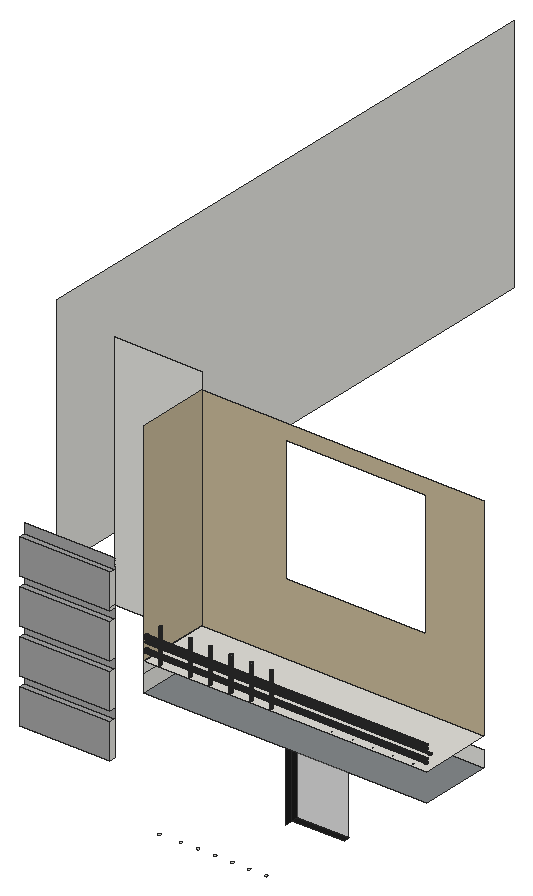
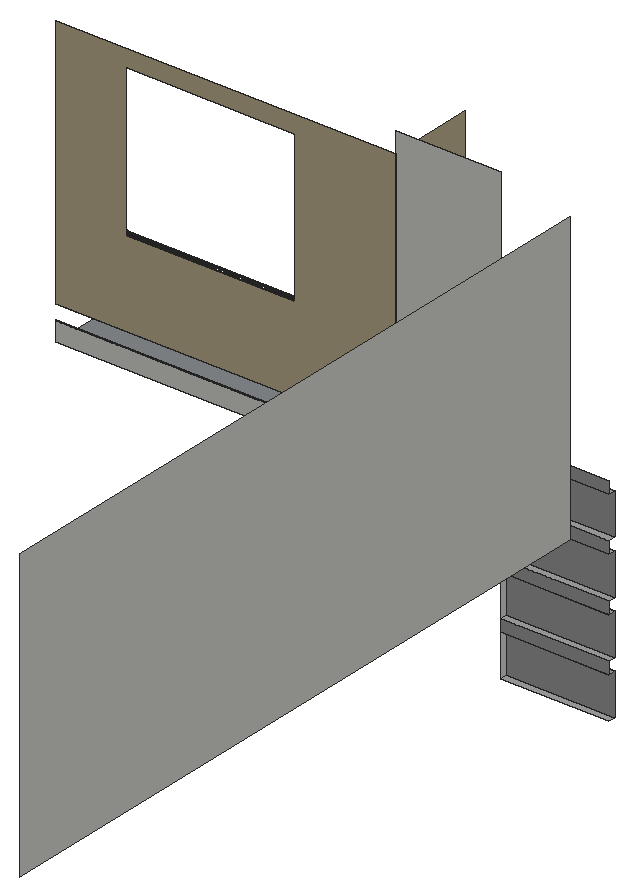
# SketchUp Ruby script. Lengths in inches.
U = 1.inch
M = Sketchup.active_model
def pt(a) = Geom::Point3d.new(a.map { |v| v * U })
def face(e, loops, mat)
  f = e.add_face(loops[0].map { |a| pt(a) })
  loops[1..].each { |l| e.add_face(l.map { |a| pt(a) }).erase! }
  f.material = f.back_material = mat if mat
  f
end
# faces: each face lists its corners as indices into pts; further lists are holes
def faces(e, pts, list, mat = nil) = list.each { |f| face(e, (f[0].is_a?(Array) ? f : [f]).map { |l| l.map { |i| pts[i] } }, mat) }
# xy, xz, yz: faces in a plane at the given z, y or x. An outline is a flat list of corners, or four numbers for a rectangle; further outlines are holes
def ring(l) = l.size == 4 ? [[l[0], l[1]], [l[2], l[1]], [l[2], l[3]], [l[0], l[3]]] : l.each_slice(2).to_a
def flat(e, list, mat, &to3) = list.each { |f| face(e, (f[0].is_a?(Array) ? f : [f]).map { |l| ring(l).map { |u, v| to3.(u, v) } }, mat) }
def xy(e, z, list, mat = nil) = flat(e, list, mat) { |x, y| [x, y, z] }
def xz(e, y, list, mat = nil) = flat(e, list, mat) { |x, z| [x, y, z] }
def yz(e, x, list, mat = nil) = flat(e, list, mat) { |y, z| [x, y, z] }
def lines(e, pts, list) = list.each { |a, b| e.add_line(pt(pts[a]), pt(pts[b])) }
# prism: a flat outline (further loops are holes) pulled along v
def prism(e, loops, v, mat = nil)
  f = face(e, loops, mat); d = Geom::Vector3d.new(v.map { |x| x * U })
  f.pushpull(f.normal.samedirection?(d) ? d.length : -d.length)
end
def box(e, o, s, mat = nil) = prism(e, [[o, [o[0] + s[0], o[1], o[2]], [o[0] + s[0], o[1] + s[1], o[2]], [o[0], o[1] + s[1], o[2]]]], [0, 0, s[2]], mat)
def at(x, y, z, deg = 0) = Geom::Transformation.translation(pt([x, y, z])) * Geom::Transformation.rotation(ORIGIN, Z_AXIS, deg.degrees)
def axes(o, x, y, z) = Geom::Transformation.new([*x, 0, *y, 0, *z, 0, *pt(o).to_a, 1])
def part(name) = M.definitions.add(name)
# library, detail: a bought-in or finely detailed component or shape, given as its bounding box
def library(name, o, s) = part(name).tap { |d| box(d.entities, o, s) }
def detail(e, o, s) = box(e.add_group.entities, o, s)
def put(e, d, t, mat = nil) = e.add_instance(d, t).tap { |i| i.material = mat if mat }
def group(e, t, mat = nil) = e.add_group.tap { |g| g.transformation = t; g.material = mat if mat }.entities
root = M.entities
M.materials.add("[0133_Gray]").color = [128, 128, 128]
M.materials.add("[Blacktop New]").color = [30, 30, 30]
M.materials.add("[Blacktop Old 01]").color = [132, 136, 139]
M.materials.add("[Marble Carrara Gold Floor Tile]").color = [225, 223, 217]
M.materials.add("[Pavers Flagstone Gray]").color = [162, 162, 162]
M.materials.add("[Quartz Light Brown]").color = [199, 184, 152]
M.materials.add("[Translucent Glass Gray]").color = [128, 128, 128]
M.materials["[Translucent Glass Gray]"].alpha = 0.5
xy(root,170.4,[[95.31,3.4,95.45,3.4,95.57,3.44,95.68,3.52,95.76,3.61,95.82,3.73,95.85,3.86,95.84,3.99,95.8,4.11,95.73,4.22,95.63,4.31,95.51,4.37,95.39,4.39,95.26,4.39,95.13,4.34,95.02,4.27,94.9375,4.18,94.88,4.06,94.85,3.93,94.86,3.8,94.9,3.68,94.97,3.57,95.07,3.48,95.1875,3.42]])
xy(root,170.77,[[106.13,3.4,106.26,3.4,106.38,3.44,106.49,3.52,106.58,3.61,106.64,3.73,106.66,3.86,106.65,3.99,106.61,4.11,106.54,4.22,106.44,4.31,106.33,4.37,106.2,4.39,106.07,4.39,105.94,4.34,105.84,4.27,105.75,4.18,105.69,4.06,105.66,3.93,105.67,3.8,105.71,3.68,105.79,3.57,105.88,3.48,106,3.42],[114.69,3.4,114.82,3.4,114.94,3.44,115.05,3.52,115.14,3.61,115.2,3.73,115.22,3.86,115.22,3.99,115.18,4.11,115.1,4.22,115.01,4.31,114.89,4.37,114.76,4.39,114.63,4.39,114.51,4.34,114.4,4.27,114.3125,4.18,114.25,4.06,114.23,3.93,114.23,3.8,114.28,3.68,114.35,3.57,114.45,3.48,114.5625,3.42],[123.25,3.4,123.38,3.4,123.51,3.44,123.62,3.52,123.7,3.61,123.76,3.73,123.79,3.86,123.78,3.99,123.74,4.11,123.67,4.22,123.57,4.31,123.45,4.37,123.32,4.39,123.19,4.39,123.07,4.34,122.96,4.27,122.875,4.18,122.82,4.06,122.79,3.93,122.8,3.8,122.84,3.68,122.91,3.57,123.01,3.48,123.125,3.42],[131.81,3.4,131.95,3.4,132.07,3.44,132.18,3.52,132.26,3.61,132.32,3.73,132.35,3.86,132.34,3.99,132.3,4.11,132.23,4.22,132.13,4.31,132.01,4.37,131.89,4.39,131.76,4.39,131.63,4.34,131.52,4.27,131.4375,4.18,131.38,4.06,131.35,3.93,131.36,3.8,131.4,3.68,131.47,3.57,131.57,3.48,131.6875,3.42],[140.38,3.4,140.51,3.4,140.63,3.44,140.74,3.52,140.83,3.61,140.89,3.73,140.91,3.86,140.9,3.99,140.86,4.11,140.79,4.22,140.69,4.31,140.58,4.37,140.45,4.39,140.32,4.39,140.19,4.34,140.09,4.27,140,4.18,139.94,4.06,139.91,3.93,139.92,3.8,139.96,3.68,140.04,3.57,140.13,3.48,140.25,3.42],
  [148.94,3.4,149.07,3.4,149.19,3.44,149.3,3.52,149.39,3.61,149.45,3.73,149.47,3.86,149.47,3.99,149.43,4.11,149.35,4.22,149.26,4.31,149.14,4.37,149.01,4.39,148.88,4.39,148.76,4.34,148.65,4.27,148.5625,4.18,148.5,4.06,148.48,3.93,148.48,3.8,148.53,3.68,148.6,3.57,148.7,3.48,148.8125,3.42]])
xy(root,171.57,[[0,36,45.0625,39]],"[Pavers Flagstone Gray]")
xy(root,176.78,[[136.06,36,162.28,39]],"[Blacktop New]")
xy(root,188.9375,[[0,36,45.0625,39]],"[Pavers Flagstone Gray]")
xy(root,193.95,[[0,36,45.0625,39]],"[Pavers Flagstone Gray]")
xy(root,211.3125,[[0,36,45.0625,39]],"[Pavers Flagstone Gray]")
xy(root,216.32,[[0,36,45.0625,39]],"[Pavers Flagstone Gray]")
xy(root,220.84,[[136.06,36,162.28,39]],"[Blacktop New]")
xy(root,232,[[88.53,3,229.62,39]],"[Blacktop Old 01]")
xy(root,233.6875,[[0,36,45.0625,39]],"[Pavers Flagstone Gray]")
xy(root,238.7,[[0,36,45.0625,39]],"[Pavers Flagstone Gray]")
xy(root,246.23,[[[88.53,3,229.62,39],[110.48,3.83,110.32,3.85,110.17,3.92,110.04,4.02,109.9375,4.15,109.875,4.3,109.85,4.46,109.875,4.62,109.9375,4.77,110.04,4.9,110.17,5,110.32,5.0625,110.48,5.08,110.64,5.0625,110.79,5,110.92,4.9,111.02,4.77,111.08,4.62,111.1,4.46,111.08,4.3,111.02,4.15,110.92,4.02,110.79,3.92,110.64,3.85],[120.6,3.83,120.44,3.85,120.29,3.92,120.16,4.02,120.0625,4.15,120,4.3,119.98,4.46,120,4.62,120.0625,4.77,120.16,4.9,120.29,5,120.44,5.0625,120.6,5.08,120.77,5.0625,120.92,5,121.05,4.9,121.15,4.77,121.21,4.62,121.23,4.46,121.21,4.3,121.15,4.15,121.05,4.02,120.92,3.92,120.77,3.85],[130.73,3.83,130.57,3.85,130.42,3.92,130.29,4.02,130.1875,4.15,130.125,4.3,130.1,4.46,130.125,4.62,130.1875,4.77,130.29,4.9,130.42,5,130.57,5.0625,130.73,5.08,130.89,5.0625,131.04,5,131.17,4.9,131.27,4.77,131.33,4.62,131.35,4.46,131.33,4.3,131.27,4.15,131.17,4.02,131.04,3.92,130.89,3.85],[140.85,3.83,140.69,3.85,140.54,3.92,140.41,4.02,140.3125,4.15,140.25,4.3,140.23,4.46,140.25,4.62,140.3125,4.77,140.41,4.9,140.54,5,140.69,5.0625,140.85,5.08,141.02,5.0625,141.17,5,141.3,4.9,141.4,4.77,141.46,4.62,141.48,4.46,141.46,4.3,141.4,4.15,141.3,4.02,141.17,3.92,141.02,3.85],[150.98,3.83,150.82,3.85,150.67,3.92,150.54,4.02,150.4375,4.15,150.375,4.3,150.35,4.46,150.375,4.62,150.4375,4.77,150.54,4.9,150.67,5,150.82,5.0625,150.98,5.08,151.14,5.0625,151.29,5,151.42,4.9,151.52,4.77,151.58,4.62,151.6,4.46,151.58,4.3,151.52,4.15,151.42,4.02,151.29,3.92,151.14,3.85],[161.1,3.83,160.94,3.85,160.79,3.92,160.66,4.02,160.5625,4.15,160.5,4.3,160.48,4.46,160.5,4.62,160.5625,4.77,160.66,4.9,160.79,5,160.94,5.0625,161.1,5.08,161.27,5.0625,161.42,5,161.55,4.9,161.65,4.77,161.71,4.62,161.73,4.46,161.71,4.3,161.65,4.15,161.55,4.02,161.42,3.92,161.27,3.85],[171.23,3.83,171.07,3.85,170.92,3.92,170.79,4.02,170.6875,4.15,170.625,4.3,170.6,4.46,170.625,4.62,170.6875,4.77,170.79,4.9,170.92,5,171.07,5.0625,171.23,5.08,171.39,5.0625,171.54,5,171.67,4.9,171.77,4.77,171.83,4.62,171.85,4.46,171.83,4.3,171.77,4.15,171.67,4.02,171.54,3.92,171.39,3.85],[181.35,3.83,181.19,3.85,181.04,3.92,180.91,4.02,180.8125,4.15,180.75,4.3,180.73,4.46,180.75,4.62,180.8125,4.77,180.91,4.9,181.04,5,181.19,5.0625,181.35,5.08,181.52,5.0625,181.67,5,181.8,4.9,181.9,4.77,181.96,4.62,181.98,4.46,181.96,4.3,181.9,4.15,181.8,4.02,181.67,3.92,181.52,3.85],[95.48,3.83,95.32,3.85,95.17,3.92,95.04,4.02,94.9375,4.15,94.875,4.3,94.85,4.46,94.875,4.62,94.9375,4.77,95.04,4.9,95.17,5,95.32,5.0625,95.48,5.08,95.64,5.0625,95.79,5,95.92,4.9,96.02,4.77,96.08,4.62,96.1,4.46,96.08,4.3,96.02,4.15,95.92,4.02,95.79,3.92,95.64,3.85],[191.48,3.83,191.32,3.85,191.17,3.92,191.04,4.02,190.9375,4.15,190.875,4.3,190.85,4.46,190.875,4.62,190.9375,4.77,191.04,4.9,191.17,5,191.32,5.0625,191.48,5.08,191.64,5.0625,191.79,5,191.92,4.9,192.02,4.77,192.08,4.62,192.1,4.46,192.08,4.3,192.02,4.15,191.92,4.02,191.79,3.92,191.64,3.85],[201.6,3.83,201.44,3.85,201.29,3.92,201.16,4.02,201.0625,4.15,201,4.3,200.98,4.46,201,4.62,201.0625,4.77,201.16,4.9,201.29,5,201.44,5.0625,201.6,5.08,201.77,5.0625,201.92,5,202.05,4.9,202.15,4.77,202.21,4.62,202.23,4.46,202.21,4.3,202.15,4.15,202.05,4.02,201.92,3.92,201.77,3.85],[211.73,3.83,211.57,3.85,211.42,3.92,211.29,4.02,211.1875,4.15,211.125,4.3,211.1,4.46,211.125,4.62,211.1875,4.77,211.29,4.9,211.42,5,211.57,5.0625,211.73,5.08,211.89,5.0625,212.04,5,212.17,4.9,212.27,4.77,212.33,4.62,212.35,4.46,212.33,4.3,212.27,4.15,212.17,4.02,212.04,3.92,211.89,3.85],[221.85,3.83,221.69,3.85,221.54,3.92,221.41,4.02,221.3125,4.15,221.25,4.3,221.23,4.46,221.25,4.62,221.3125,4.77,221.41,4.9,221.54,5,221.69,5.0625,221.85,5.08,222.02,5.0625,222.17,5,222.3,4.9,222.4,4.77,222.46,4.62,222.48,4.46,222.46,4.3,222.4,4.15,222.3,4.02,222.17,3.92,222.02,3.85]]],"[Marble Carrara Gold Floor Tile]")
xy(root,256.0625,[[0,36,45.0625,39]],"[Pavers Flagstone Gray]")
xz(root,36,[[0,171.57,45.0625,188.9375],[0,193.95,45.0625,211.3125],[0,216.32,45.0625,233.6875],[0,238.7,45.0625,256.0625]],"[Pavers Flagstone Gray]")
xz(root,39,[[88.53,232,229.62,240],[45.0625,240,88.53,360],[88.53,240,229.62,240.1875]])
xz(root,39,[[0,188.9375,45.0625,193.95],[0,211.3125,45.0625,216.32],[0,233.6875,45.0625,238.7],[0,256.0625,45.0625,261.07]],"[Pavers Flagstone Gray]")
xz(root,39,[[[88.53,246.23,229.62,351.5625],[130.59,281.71,200.77,344.28]]],"[Quartz Light Brown]")
xz(root,39,[[136.06,176.78,162.28,220.84]],"[Translucent Glass Gray]")
yz(root,9,[[48,240,333.4375,360]])
yz(root,45.0625,[[36,171.57,39,188.9375],[36,193.95,39,211.3125],[36,216.32,39,233.6875],[36,238.7,39,240],[36,240,39,256.0625]])
yz(root,88.53,[[3,232,39,240.1875],[3,240.1875,39,246.23]])
yz(root,88.53,[[[3,246.23,39,351.5625],[3.53,257.33,3.43,257.34,3.34,257.375,3.26,257.43,3.2,257.51,3.16,257.6,3.15,257.7,3.16,257.8,3.2,257.89,3.26,257.97,3.34,258.02,3.43,258.0625,3.53,258.08,3.625,258.0625,3.71,258.02,3.79,257.97,3.85,257.89,3.89,257.8,3.9,257.7,3.89,257.6,3.85,257.51,3.79,257.43,3.71,257.375,3.625,257.34],[3.53,258.89,3.43,258.9,3.34,258.9375,3.26,259,3.2,259.08,3.16,259.17,3.15,259.26,3.16,259.36,3.2,259.45,3.26,259.53,3.34,259.59,3.43,259.625,3.53,259.64,3.625,259.625,3.71,259.59,3.79,259.53,3.85,259.45,3.89,259.36,3.9,259.26,3.89,259.17,3.85,259.08,3.79,259,3.71,258.9375,3.625,258.9],[3.53,260.45,3.43,260.46,3.34,260.5,3.26,260.56,3.2,260.64,3.16,260.73,3.15,260.83,3.16,260.92,3.2,261.01,3.26,261.09,3.34,261.15,3.43,261.1875,3.53,261.2,3.625,261.1875,3.71,261.15,3.79,261.09,3.85,261.01,3.89,260.92,3.9,260.83,3.89,260.73,3.85,260.64,3.79,260.56,3.71,260.5,3.625,260.46],[3.53,262.01,3.43,262.03,3.34,262.0625,3.26,262.12,3.2,262.2,3.16,262.29,3.15,262.39,3.16,262.48,3.2,262.58,3.26,262.65,3.34,262.71,3.43,262.75,3.53,262.76,3.625,262.75,3.71,262.71,3.79,262.65,3.85,262.58,3.89,262.48,3.9,262.39,3.89,262.29,3.85,262.2,3.79,262.12,3.71,262.0625,3.625,262.03],[3.53,255.76,3.43,255.78,3.34,255.8125,3.26,255.87,3.2,255.95,3.16,256.04,3.15,256.14,3.16,256.23,3.2,256.33,3.26,256.4,3.34,256.46,3.43,256.5,3.53,256.51,3.625,256.5,3.71,256.46,3.79,256.4,3.85,256.33,3.89,256.23,3.9,256.14,3.89,256.04,3.85,255.95,3.79,255.87,3.71,255.8125,3.625,255.78],[3.53,247.95,3.43,247.96,3.34,248,3.26,248.06,3.2,248.14,3.16,248.23,3.15,248.33,3.16,248.42,3.2,248.51,3.26,248.59,3.34,248.65,3.43,248.6875,3.53,248.7,3.625,248.6875,3.71,248.65,3.79,248.59,3.85,248.51,3.89,248.42,3.9,248.33,3.89,248.23,3.85,248.14,3.79,248.06,3.71,248,3.625,247.96],[3.53,249.51,3.43,249.53,3.34,249.5625,3.26,249.62,3.2,249.7,3.16,249.79,3.15,249.89,3.16,249.98,3.2,250.08,3.26,250.15,3.34,250.21,3.43,250.25,3.53,250.26,3.625,250.25,3.71,250.21,3.79,250.15,3.85,250.08,3.89,249.98,3.9,249.89,3.89,249.79,3.85,249.7,3.79,249.62,3.71,249.5625,3.625,249.53],[3.53,251.08,3.43,251.09,3.34,251.125,3.26,251.18,3.2,251.26,3.16,251.35,3.15,251.45,3.16,251.55,3.2,251.64,3.26,251.72,3.34,251.77,3.43,251.8125,3.53,251.83,3.625,251.8125,3.71,251.77,3.79,251.72,3.85,251.64,3.89,251.55,3.9,251.45,3.89,251.35,3.85,251.26,3.79,251.18,3.71,251.125,3.625,251.09],[3.53,252.64,3.43,252.65,3.34,252.6875,3.26,252.75,3.2,252.83,3.16,252.92,3.15,253.01,3.16,253.11,3.2,253.2,3.26,253.28,3.34,253.34,3.43,253.375,3.53,253.39,3.625,253.375,3.71,253.34,3.79,253.28,3.85,253.2,3.89,253.11,3.9,253.01,3.89,252.92,3.85,252.83,3.79,252.75,3.71,252.6875,3.625,252.65],[3.53,254.2,3.43,254.21,3.34,254.25,3.26,254.31,3.2,254.39,3.16,254.48,3.15,254.58,3.16,254.67,3.2,254.76,3.26,254.84,3.34,254.9,3.43,254.9375,3.53,254.95,3.625,254.9375,3.71,254.9,3.79,254.84,3.85,254.76,3.89,254.67,3.9,254.58,3.89,254.48,3.85,254.39,3.79,254.31,3.71,254.25,3.625,254.21]]],"[Quartz Light Brown]")
yz(root,133.06,[[36,173.78,39,223.84]],"[Blacktop New]")
yz(root,136.06,[[36,176.78,39,220.84]],"[Blacktop New]")
p = [[95.32,3.85,246.23],[95.48,3.83,246.23],[95.48,3.83,263.16],[95.32,3.85,263.16],[95.64,3.85,246.23],[95.64,3.85,263.16],
  [110.32,3.85,246.23],[110.48,3.83,246.23],[110.48,3.83,263.16],[110.32,3.85,263.16],[110.64,3.85,246.23],[110.64,3.85,263.16],
  [120.44,3.85,246.23],[120.6,3.83,246.23],[120.6,3.83,263.16],[120.44,3.85,263.16],[120.77,3.85,246.23],[120.77,3.85,263.16],
  [130.57,3.85,246.23],[130.73,3.83,246.23],[130.73,3.83,263.16],[130.57,3.85,263.16],[130.89,3.85,246.23],[130.89,3.85,263.16],
  [140.69,3.85,246.23],[140.85,3.83,246.23],[140.85,3.83,263.16],[140.69,3.85,263.16],[141.02,3.85,246.23],[141.02,3.85,263.16],
  [150.82,3.85,246.23],[150.98,3.83,246.23],[150.98,3.83,263.16],[150.82,3.85,263.16],[151.14,3.85,246.23],[151.14,3.85,263.16],
  [95.04,4.02,246.23],[95.17,3.92,246.23],[95.17,3.92,263.16],[95.04,4.02,263.16],[95.79,3.92,246.23],[95.79,3.92,263.16],
  [95.92,4.02,246.23],[95.92,4.02,263.16],[110.04,4.02,246.23],[110.17,3.92,246.23],[110.17,3.92,263.16],[110.04,4.02,263.16],
  [110.79,3.92,246.23],[110.79,3.92,263.16],[110.92,4.02,246.23],[110.92,4.02,263.16],[120.16,4.02,246.23],[120.29,3.92,246.23],
  [120.29,3.92,263.16],[120.16,4.02,263.16],[120.92,3.92,246.23],[120.92,3.92,263.16],[121.05,4.02,246.23],[121.05,4.02,263.16],
  [130.29,4.02,246.23],[130.42,3.92,246.23],[130.42,3.92,263.16],[130.29,4.02,263.16],[131.04,3.92,246.23],[131.04,3.92,263.16],
  [131.17,4.02,246.23],[131.17,4.02,263.16],[140.41,4.02,246.23],[140.54,3.92,246.23],[140.54,3.92,263.16],[140.41,4.02,263.16],
  [141.17,3.92,246.23],[141.17,3.92,263.16],[141.3,4.02,246.23],[141.3,4.02,263.16],[150.54,4.02,246.23],[150.67,3.92,246.23],
  [150.67,3.92,263.16],[150.54,4.02,263.16],[151.29,3.92,246.23],[151.29,3.92,263.16],[151.42,4.02,246.23],[151.42,4.02,263.16],
  [94.9375,4.15,246.23],[94.9375,4.15,263.16],[96.02,4.15,246.23],[96.02,4.15,263.16],[109.9375,4.15,246.23],[109.9375,4.15,263.16],
  [111.02,4.15,246.23],[111.02,4.15,263.16],[120.0625,4.15,246.23],[120.0625,4.15,263.16],[121.15,4.15,246.23],[121.15,4.15,263.16],
  [130.1875,4.15,246.23],[130.1875,4.15,263.16],[131.27,4.15,246.23],[131.27,4.15,263.16],[140.3125,4.15,246.23],[140.3125,4.15,263.16],
  [141.4,4.15,246.23],[141.4,4.15,263.16],[150.4375,4.15,246.23],[150.4375,4.15,263.16],[151.52,4.15,246.23],[151.52,4.15,263.16],
  [94.875,4.3,246.23],[94.875,4.3,263.16],[96.08,4.3,246.23],[96.08,4.3,263.16],[109.875,4.3,246.23],[109.875,4.3,263.16],
  [111.08,4.3,246.23],[111.08,4.3,263.16],[120,4.3,246.23],[120,4.3,263.16],[121.21,4.3,246.23],[121.21,4.3,263.16],
  [130.125,4.3,246.23],[130.125,4.3,263.16],[131.33,4.3,246.23],[131.33,4.3,263.16],[140.25,4.3,246.23],[140.25,4.3,263.16],
  [141.46,4.3,246.23],[141.46,4.3,263.16],[150.375,4.3,246.23],[150.375,4.3,263.16],[151.58,4.3,246.23],[151.58,4.3,263.16],
  [94.85,4.46,246.23],[94.85,4.46,263.16],[96.1,4.46,246.23],[96.1,4.46,263.16],[109.85,4.46,246.23],[109.85,4.46,263.16],
  [111.1,4.46,246.23],[111.1,4.46,263.16],[119.98,4.46,246.23],[119.98,4.46,263.16],[121.23,4.46,246.23],[121.23,4.46,263.16],
  [130.1,4.46,246.23],[130.1,4.46,263.16],[131.35,4.46,246.23],[131.35,4.46,263.16],[140.23,4.46,246.23],[140.23,4.46,263.16],
  [141.48,4.46,246.23],[141.48,4.46,263.16],[150.35,4.46,246.23],[150.35,4.46,263.16],[151.6,4.46,246.23],[151.6,4.46,263.16],
  [94.875,4.62,246.23],[94.875,4.62,263.16],[96.08,4.62,246.23],[96.08,4.62,263.16],[109.875,4.62,246.23],[109.875,4.62,263.16],
  [111.08,4.62,246.23],[111.08,4.62,263.16],[120,4.62,246.23],[120,4.62,263.16],[121.21,4.62,246.23],[121.21,4.62,263.16],
  [130.125,4.62,246.23],[130.125,4.62,263.16],[131.33,4.62,246.23],[131.33,4.62,263.16],[140.25,4.62,246.23],[140.25,4.62,263.16],
  [141.46,4.62,246.23],[141.46,4.62,263.16],[150.375,4.62,246.23],[150.375,4.62,263.16],[151.58,4.62,246.23],[151.58,4.62,263.16],
  [94.9375,4.77,246.23],[94.9375,4.77,263.16],[96.02,4.77,246.23],[96.02,4.77,263.16],[109.9375,4.77,246.23],[109.9375,4.77,263.16],
  [111.02,4.77,246.23],[111.02,4.77,263.16],[120.0625,4.77,246.23],[120.0625,4.77,263.16],[121.15,4.77,246.23],[121.15,4.77,263.16],
  [130.1875,4.77,246.23],[130.1875,4.77,263.16],[131.27,4.77,246.23],[131.27,4.77,263.16],[140.3125,4.77,246.23],[140.3125,4.77,263.16],
  [141.4,4.77,246.23],[141.4,4.77,263.16],[150.4375,4.77,246.23],[150.4375,4.77,263.16],[151.52,4.77,246.23],[151.52,4.77,263.16],
  [95.04,4.9,246.23],[95.04,4.9,263.16],[95.92,4.9,246.23],[95.92,4.9,263.16],[110.04,4.9,246.23],[110.04,4.9,263.16],
  [110.92,4.9,246.23],[110.92,4.9,263.16],[120.16,4.9,246.23],[120.16,4.9,263.16],[121.05,4.9,246.23],[121.05,4.9,263.16],
  [130.29,4.9,246.23],[130.29,4.9,263.16],[131.17,4.9,246.23],[131.17,4.9,263.16],[140.41,4.9,246.23],[140.41,4.9,263.16],
  [141.3,4.9,246.23],[141.3,4.9,263.16],[150.54,4.9,246.23],[150.54,4.9,263.16],[151.42,4.9,246.23],[151.42,4.9,263.16],
  [95.17,5,246.23],[95.17,5,263.16],[95.79,5,246.23],[95.79,5,263.16],[110.17,5,246.23],[110.17,5,263.16],
  [110.79,5,246.23],[110.79,5,263.16],[120.29,5,246.23],[120.29,5,263.16],[120.92,5,246.23],[120.92,5,263.16],
  [130.42,5,246.23],[130.42,5,263.16],[131.04,5,246.23],[131.04,5,263.16],[140.54,5,246.23],[140.54,5,263.16],
  [141.17,5,246.23],[141.17,5,263.16],[150.67,5,246.23],[150.67,5,263.16],[151.29,5,246.23],[151.29,5,263.16],
  [95.32,5.0625,246.23],[95.32,5.0625,263.16],[95.64,5.0625,246.23],[95.64,5.0625,263.16],[110.32,5.0625,246.23],[110.32,5.0625,263.16],
  [110.64,5.0625,246.23],[110.64,5.0625,263.16],[120.44,5.0625,246.23],[120.44,5.0625,263.16],[120.77,5.0625,246.23],[120.77,5.0625,263.16],
  [130.57,5.0625,246.23],[130.57,5.0625,263.16],[130.89,5.0625,246.23],[130.89,5.0625,263.16],[140.69,5.0625,246.23],[140.69,5.0625,263.16],
  [141.02,5.0625,246.23],[141.02,5.0625,263.16],[150.82,5.0625,246.23],[150.82,5.0625,263.16],[151.14,5.0625,246.23],[151.14,5.0625,263.16],
  [95.48,5.08,246.23],[95.48,5.08,263.16],[110.48,5.08,246.23],[110.48,5.08,263.16],[120.6,5.08,246.23],[120.6,5.08,263.16],
  [130.73,5.08,246.23],[130.73,5.08,263.16],[140.85,5.08,246.23],[140.85,5.08,263.16],[150.98,5.08,246.23],[150.98,5.08,263.16],
  [88.53,3.34,249.5625],[88.53,3.43,249.53],[229.62,3.43,249.53],[229.62,3.34,249.5625],[88.53,3.53,249.51],[229.62,3.53,249.51],
  [88.53,3.625,249.53],[229.62,3.625,249.53],[88.53,3.71,249.5625],[229.62,3.71,249.5625],[88.53,3.2,249.7],[88.53,3.26,249.62],
  [229.62,3.26,249.62],[229.62,3.2,249.7],[88.53,3.79,249.62],[229.62,3.79,249.62],[88.53,3.85,249.7],[229.62,3.85,249.7],
  [88.53,3.16,249.79],[229.62,3.16,249.79],[88.53,3.89,249.79],[229.62,3.89,249.79],[88.53,3.15,249.89],[229.62,3.15,249.89],
  [88.53,3.9,249.89],[229.62,3.9,249.89],[88.53,3.16,249.98],[229.62,3.16,249.98],[88.53,3.89,249.98],[229.62,3.89,249.98],
  [88.53,3.2,250.08],[229.62,3.2,250.08],[88.53,3.85,250.08],[229.62,3.85,250.08],[88.53,3.26,250.15],[229.62,3.26,250.15],
  [88.53,3.79,250.15],[229.62,3.79,250.15],[88.53,3.34,250.21],[229.62,3.34,250.21],[88.53,3.43,250.25],[229.62,3.43,250.25],
  [88.53,3.53,250.26],[229.62,3.53,250.26],[88.53,3.625,250.25],[229.62,3.625,250.25],[88.53,3.71,250.21],[229.62,3.71,250.21],
  [88.53,3.34,251.125],[88.53,3.43,251.09],[229.62,3.43,251.09],[229.62,3.34,251.125],[88.53,3.26,251.18],[229.62,3.26,251.18],
  [88.53,3.53,251.08],[229.62,3.53,251.08],[88.53,3.625,251.09],[229.62,3.625,251.09],[88.53,3.71,251.125],[229.62,3.71,251.125],
  [88.53,3.79,251.18],[229.62,3.79,251.18],[88.53,3.2,251.26],[229.62,3.2,251.26],[88.53,3.85,251.26],[229.62,3.85,251.26],
  [88.53,3.16,251.35],[229.62,3.16,251.35],[88.53,3.89,251.35],[229.62,3.89,251.35],[88.53,3.15,251.45],[229.62,3.15,251.45],
  [88.53,3.9,251.45],[229.62,3.9,251.45],[88.53,3.16,251.55],[229.62,3.16,251.55],[88.53,3.2,251.64],[229.62,3.2,251.64],
  [88.53,3.89,251.55],[229.62,3.89,251.55],[88.53,3.85,251.64],[229.62,3.85,251.64],[88.53,3.26,251.72],[229.62,3.26,251.72],
  [88.53,3.79,251.72],[229.62,3.79,251.72],[88.53,3.34,251.77],[229.62,3.34,251.77],[88.53,3.71,251.77],[229.62,3.71,251.77],
  [88.53,3.43,251.8125],[229.62,3.43,251.8125],[88.53,3.53,251.83],[229.62,3.53,251.83],[88.53,3.625,251.8125],[229.62,3.625,251.8125],
  [88.53,3.34,254.25],[88.53,3.43,254.21],[231.78,3.43,254.21],[231.78,3.34,254.25],[88.53,3.53,254.2],[231.78,3.53,254.2],
  [88.53,3.625,254.21],[231.78,3.625,254.21],[88.53,3.71,254.25],[231.78,3.71,254.25],[88.53,3.2,254.39],[88.53,3.26,254.31],
  [231.78,3.26,254.31],[231.78,3.2,254.39],[88.53,3.79,254.31],[231.78,3.79,254.31],[88.53,3.85,254.39],[231.78,3.85,254.39],
  [88.53,3.16,254.48],[231.78,3.16,254.48],[88.53,3.89,254.48],[231.78,3.89,254.48],[88.53,3.15,254.58],[231.78,3.15,254.58],
  [88.53,3.9,254.58],[231.78,3.9,254.58],[88.53,3.16,254.67],[231.78,3.16,254.67],[88.53,3.89,254.67],[231.78,3.89,254.67],
  [88.53,3.2,254.76],[231.78,3.2,254.76],[88.53,3.85,254.76],[231.78,3.85,254.76],[88.53,3.34,255.8125],[88.53,3.43,255.78],
  [229.85,3.43,255.78],[229.85,3.34,255.8125],[88.53,3.26,255.87],[229.85,3.26,255.87],[88.53,3.53,255.76],[229.85,3.53,255.76],
  [88.53,3.625,255.78],[229.85,3.625,255.78],[88.53,3.71,255.8125],[229.85,3.71,255.8125],[88.53,3.79,255.87],[229.85,3.79,255.87],
  [88.53,3.2,255.95],[229.85,3.2,255.95],[88.53,3.85,255.95],[229.85,3.85,255.95],[88.53,3.16,256.04],[229.85,3.16,256.04],
  [88.53,3.15,256.14],[229.85,3.15,256.14],[88.53,3.89,256.04],[229.85,3.89,256.04],[88.53,3.9,256.14],[229.85,3.9,256.14],
  [88.53,3.16,256.23],[229.85,3.16,256.23],[88.53,3.89,256.23],[229.85,3.89,256.23],[88.53,3.2,256.33],[229.85,3.2,256.33],
  [88.53,3.85,256.33],[229.85,3.85,256.33],[88.53,3.26,256.4],[229.85,3.26,256.4],[88.53,3.79,256.4],[229.85,3.79,256.4],
  [88.53,3.34,256.46],[229.85,3.34,256.46],[88.53,3.71,256.46],[229.85,3.71,256.46],[88.53,3.43,256.5],[229.85,3.43,256.5],
  [88.53,3.53,256.51],[229.85,3.53,256.51],[88.53,3.625,256.5],[229.85,3.625,256.5],[88.53,3.34,257.375],[88.53,3.43,257.34],
  [229.62,3.43,257.34],[229.62,3.34,257.375],[88.53,3.53,257.33],[229.62,3.53,257.33],[88.53,3.625,257.34],[229.62,3.625,257.34],
  [88.53,3.71,257.375],[229.62,3.71,257.375],[88.53,3.2,257.51],[88.53,3.26,257.43],[229.62,3.26,257.43],[229.62,3.2,257.51],
  [88.53,3.79,257.43],[229.62,3.79,257.43],[88.53,3.85,257.51],[229.62,3.85,257.51],[88.53,3.16,257.6],[229.62,3.16,257.6],
  [88.53,3.89,257.6],[229.62,3.89,257.6],[88.53,3.15,257.7],[229.62,3.15,257.7],[88.53,3.9,257.7],[229.62,3.9,257.7],
  [88.53,3.16,257.8],[229.62,3.16,257.8],[88.53,3.89,257.8],[229.62,3.89,257.8],[88.53,3.2,257.89],[229.62,3.2,257.89],
  [88.53,3.85,257.89],[229.62,3.85,257.89],[88.53,3.26,257.97],[229.62,3.26,257.97],[88.53,3.79,257.97],[229.62,3.79,257.97],
  [88.53,3.34,258.02],[229.62,3.34,258.02],[88.53,3.43,258.0625],[229.62,3.43,258.0625],[88.53,3.71,258.02],[88.53,3.625,258.0625],
  [229.62,3.625,258.0625],[229.62,3.71,258.02],[88.53,3.53,258.08],[229.62,3.53,258.08]]
faces(root,p,[[0,1,2,3],[1,4,5,2],[6,7,8,9],[7,10,11,8],[12,13,14,15],[13,16,17,14],[18,19,20,21],[19,22,23,20],
  [24,25,26,27],[25,28,29,26],[30,31,32,33],[31,34,35,32],[36,37,38,39],[37,0,3,38],[4,40,41,5],[40,42,43,41],
  [44,45,46,47],[45,6,9,46],[10,48,49,11],[48,50,51,49],[52,53,54,55],[53,12,15,54],[16,56,57,17],[56,58,59,57],
  [60,61,62,63],[61,18,21,62],[22,64,65,23],[64,66,67,65],[68,69,70,71],[69,24,27,70],[28,72,73,29],[72,74,75,73],
  [76,77,78,79],[77,30,33,78],[34,80,81,35],[80,82,83,81],[84,36,39,85],[42,86,87,43],[88,44,47,89],[50,90,91,51],
  [92,52,55,93],[58,94,95,59],[96,60,63,97],[66,98,99,67],[100,68,71,101],[74,102,103,75],[104,76,79,105],[82,106,107,83],
  [108,84,85,109],[86,110,111,87],[112,88,89,113],[90,114,115,91],[116,92,93,117],[94,118,119,95],[120,96,97,121],[98,122,123,99],
  [124,100,101,125],[102,126,127,103],[128,104,105,129],[106,130,131,107],[132,108,109,133],[110,134,135,111],[136,112,113,137],[114,138,139,115],
  [140,116,117,141],[118,142,143,119],[144,120,121,145],[122,146,147,123],[148,124,125,149],[126,150,151,127],[152,128,129,153],[130,154,155,131],
  [156,132,133,157],[134,158,159,135],[160,136,137,161],[138,162,163,139],[164,140,141,165],[142,166,167,143],[168,144,145,169],[146,170,171,147],
  [172,148,149,173],[150,174,175,151],[176,152,153,177],[154,178,179,155],[180,156,157,181],[158,182,183,159],[184,160,161,185],[162,186,187,163],
  [188,164,165,189],[166,190,191,167],[192,168,169,193],[170,194,195,171],[196,172,173,197],[174,198,199,175],[200,176,177,201],[178,202,203,179],
  [204,180,181,205],[182,206,207,183],[208,184,185,209],[186,210,211,187],[212,188,189,213],[190,214,215,191],[216,192,193,217],[194,218,219,195],
  [220,196,197,221],[198,222,223,199],[224,200,201,225],[202,226,227,203],[228,204,205,229],[206,230,231,207],[232,208,209,233],[210,234,235,211],
  [236,212,213,237],[214,238,239,215],[240,216,217,241],[218,242,243,219],[244,220,221,245],[222,246,247,223],[248,224,225,249],[226,250,251,227],
  [252,228,229,253],[230,254,255,231],[256,232,233,257],[234,258,259,235],[260,236,237,261],[238,262,263,239],[264,240,241,265],[242,266,267,243],
  [268,244,245,269],[246,270,271,247],[272,248,249,273],[250,274,275,251],[276,252,253,277],[254,276,277,255],[278,256,257,279],[258,278,279,259],
  [280,260,261,281],[262,280,281,263],[282,264,265,283],[266,282,283,267],[284,268,269,285],[270,284,285,271],[286,272,273,287],[274,286,287,275],
  [288,289,290,291],[289,292,293,290],[292,294,295,293],[294,296,297,295],[298,299,300,301],[299,288,291,300],[296,302,303,297],[302,304,305,303],
  [306,298,301,307],[304,308,309,305],[310,306,307,311],[308,312,313,309],[314,310,311,315],[312,316,317,313],[318,314,315,319],[316,320,321,317],
  [322,318,319,323],[320,324,325,321],[326,322,323,327],[328,326,327,329],[330,328,329,331],[332,330,331,333],[334,332,333,335],[324,334,335,325],
  [336,337,338,339],[340,336,339,341],[337,342,343,338],[342,344,345,343],[344,346,347,345],[346,348,349,347],[350,340,341,351],[348,352,353,349],
  [354,350,351,355],[352,356,357,353],[358,354,355,359],[356,360,361,357],[362,358,359,363],[364,362,363,365],[360,366,367,361],[366,368,369,367],
  [370,364,365,371],[368,372,373,369],[374,370,371,375],[372,376,377,373],[378,374,375,379],[380,378,379,381],[382,380,381,383],[376,382,383,377],
  [384,385,386,387],[385,388,389,386],[388,390,391,389],[390,392,393,391],[394,395,396,397],[395,384,387,396],[392,398,399,393],[398,400,401,399],
  [402,394,397,403],[400,404,405,401],[406,402,403,407],[404,408,409,405],[410,406,407,411],[408,412,413,409],[414,410,411,415],[412,416,417,413],
  [418,419,420,421],[422,418,421,423],[419,424,425,420],[424,426,427,425],[426,428,429,427],[428,430,431,429],[432,422,423,433],[430,434,435,431],
  [436,432,433,437],[438,436,437,439],[434,440,441,435],[440,442,443,441],[444,438,439,445],[442,446,447,443],[448,444,445,449],[446,450,451,447],
  [452,448,449,453],[450,454,455,451],[456,452,453,457],[454,458,459,455],[460,456,457,461],[462,460,461,463],[464,462,463,465],[458,464,465,459],
  [466,467,468,469],[467,470,471,468],[470,472,473,471],[472,474,475,473],[476,477,478,479],[477,466,469,478],[474,480,481,475],[480,482,483,481],
  [484,476,479,485],[482,486,487,483],[488,484,485,489],[486,490,491,487],[492,488,489,493],[490,494,495,491],[496,492,493,497],[494,498,499,495],
  [500,496,497,501],[498,502,503,499],[504,500,501,505],[506,504,505,507],[508,509,510,511],[502,508,511,503],[512,506,507,513],[509,512,513,510]],"[0133_Gray]")
